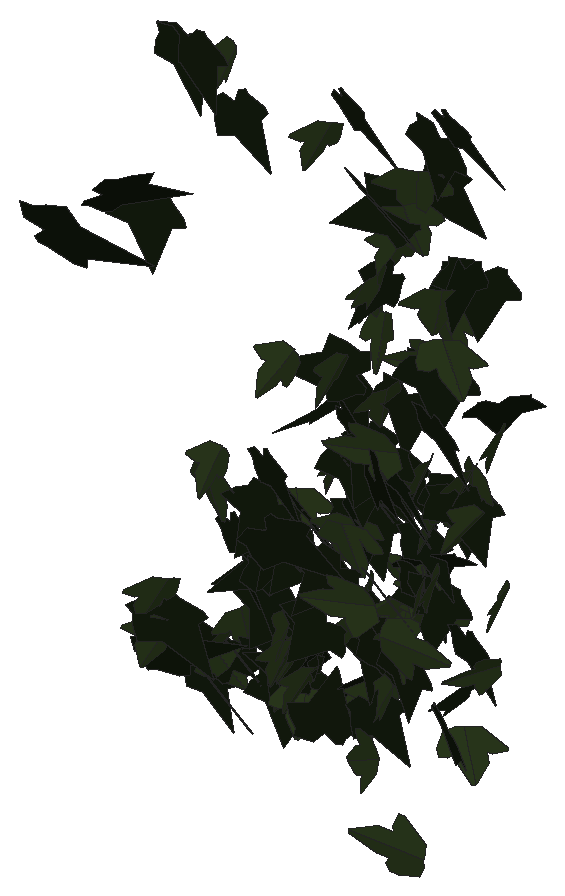
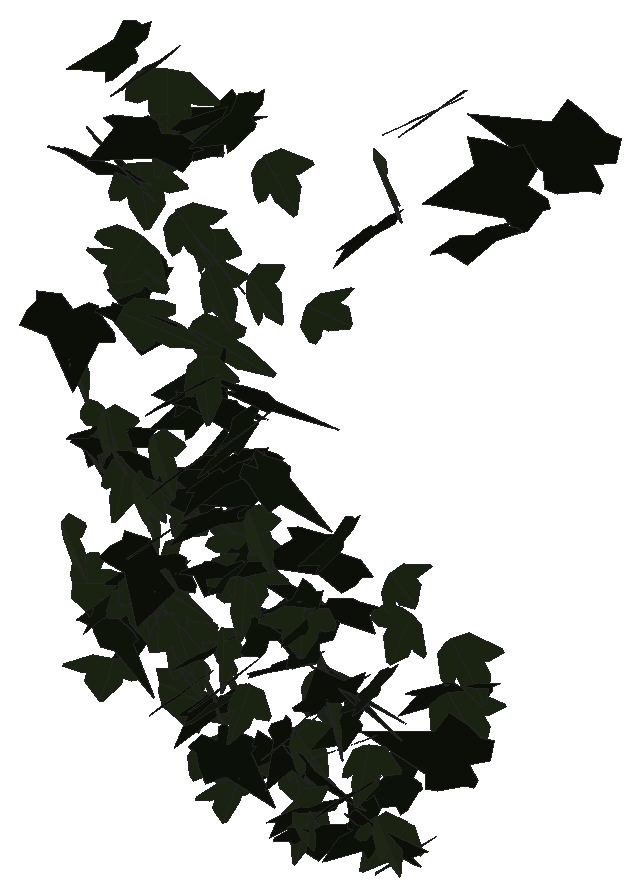
# SketchUp Ruby script. Lengths in inches.
U = 1.inch
M = Sketchup.active_model
def pt(a) = Geom::Point3d.new(a.map { |v| v * U })
def face(e, loops, mat)
  f = e.add_face(loops[0].map { |a| pt(a) })
  loops[1..].each { |l| e.add_face(l.map { |a| pt(a) }).erase! }
  f.material = f.back_material = mat if mat
  f
end
# faces: each face lists its corners as indices into pts; further lists are holes
def faces(e, pts, list, mat = nil) = list.each { |f| face(e, (f[0].is_a?(Array) ? f : [f]).map { |l| l.map { |i| pts[i] } }, mat) }
# xy, xz, yz: faces in a plane at the given z, y or x. An outline is a flat list of corners, or four numbers for a rectangle; further outlines are holes
def ring(l) = l.size == 4 ? [[l[0], l[1]], [l[2], l[1]], [l[2], l[3]], [l[0], l[3]]] : l.each_slice(2).to_a
def flat(e, list, mat, &to3) = list.each { |f| face(e, (f[0].is_a?(Array) ? f : [f]).map { |l| ring(l).map { |u, v| to3.(u, v) } }, mat) }
def xy(e, z, list, mat = nil) = flat(e, list, mat) { |x, y| [x, y, z] }
def xz(e, y, list, mat = nil) = flat(e, list, mat) { |x, z| [x, y, z] }
def yz(e, x, list, mat = nil) = flat(e, list, mat) { |y, z| [x, y, z] }
def lines(e, pts, list) = list.each { |a, b| e.add_line(pt(pts[a]), pt(pts[b])) }
# prism: a flat outline (further loops are holes) pulled along v
def prism(e, loops, v, mat = nil)
  f = face(e, loops, mat); d = Geom::Vector3d.new(v.map { |x| x * U })
  f.pushpull(f.normal.samedirection?(d) ? d.length : -d.length)
end
def box(e, o, s, mat = nil) = prism(e, [[o, [o[0] + s[0], o[1], o[2]], [o[0] + s[0], o[1] + s[1], o[2]], [o[0], o[1] + s[1], o[2]]]], [0, 0, s[2]], mat)
def at(x, y, z, deg = 0) = Geom::Transformation.translation(pt([x, y, z])) * Geom::Transformation.rotation(ORIGIN, Z_AXIS, deg.degrees)
def axes(o, x, y, z) = Geom::Transformation.new([*x, 0, *y, 0, *z, 0, *pt(o).to_a, 1])
def part(name) = M.definitions.add(name)
# library, detail: a bought-in or finely detailed component or shape, given as its bounding box
def library(name, o, s) = part(name).tap { |d| box(d.entities, o, s) }
def detail(e, o, s) = box(e.add_group.entities, o, s)
def put(e, d, t, mat = nil) = e.add_instance(d, t).tap { |i| i.material = mat if mat }
def group(e, t, mat = nil) = e.add_group.tap { |g| g.transformation = t; g.material = mat if mat }.entities
root = M.entities
M.materials.add("1026 AP 7946 SUNNY SIDE UP").color = [254, 231, 186]
M.materials.add("efeu1").color = [18, 25, 13]
M.materials.add("efeu2").color = [43, 57, 29]
c1 = part("ivyleaf_10")
p = [[0,0.5,-0.03],[-0.0625,2.02,-0.43],[-0.19,2.01,-0.46],[-0.54,1.05,-0.29],[-0.52,0.625,-0.18],[-0.83,0.76,-0.28],
  [-1.16,0.64,-0.33],[-1.15,0.33,-0.24],[-0.77,-0.39,0.02],[-0.3,-0.51,0.16],[0.04,-0.48,0.23],[-0.02,2.01,-0.4375],
  [-0.06,2.01,-0.43],[0.04,-0.49,0.23],[0.67,-0.49,0.14],[1.38,0.36,-0.2],[1.375,0.51,-0.24],[0.81,0.65,-0.19],
  [0.62,0.59,-0.15],[0.6,1.09,-0.28],[0.5,1.23,-0.31]]
faces(c1.entities,p,[[0,1,2,3,4,5,6,7,8,9,10],[11,12,0,13,14,15,16,17,18,19,20]],"efeu2")
c2 = part("ivyleaf_9")
p = [[1.54,2.16,1.25],[1.36,2.04,1.19],[-0.21,0.99,0.68],[-0.71,1.11,0.82],[-0.85,0.86,0.67],[-0.8,0.17,0.21],
  [-0.9,-0.01,0.1],[-0.67,-0.16,-0.02],[-0.08,-0.08,-0.05],[-0.03,-0.6,-0.4],[0.65,-0.88,-0.66],[0.83,-0.6,-0.49],
  [1.29,-0.42,-0.43],[1.8125,-0.07,-0.26],[1.21,0.44,0.15]]
faces(c2.entities,p,[[0,1,2,3,4,5,6,7,8,9,10,11,12,13,14]],"efeu1")
put(root,c1,axes([100.4,212.9375,280.08],[0.04345,-0.30572,0.04856],[-0.00086,-0.04912,-0.31648],[0.48681,0.0272,-0.0049]),"1026 AP 7946 SUNNY SIDE UP")
put(root,c1,axes([100.4,212.96,290.27],[0.30495,-0.28987,0.00995],[-0.00585,-0.01609,-0.35918],[0.45611,0.1936,-0.01126]),"1026 AP 7946 SUNNY SIDE UP")
put(root,c2,axes([100.73,212.63,279.72],[0.02636,0.13505,0.28405],[-0.34904,0.19485,-0.0912],[-0.36179,-0.17815,0.10868]),"1026 AP 7946 SUNNY SIDE UP")
put(root,c2,axes([100.32,211.1,288.47],[-0.12264,-0.34292,-0.04501],[0.01448,0.04072,-0.36206],[0.543,-0.07854,-0.00051]),"1026 AP 7946 SUNNY SIDE UP")
put(root,c2,axes([100.25,212.03,290.83],[0.05539,-0.34177,0.02697],[-0.01052,-0.03036,-0.36785],[0.58225,0.03196,-0.00921]),"1026 AP 7946 SUNNY SIDE UP")
put(root,c1,axes([100.46,212.44,283.04],[-0.46721,0.14937,-0.03435],[0.03162,-0.03683,-0.33483],[-0.25814,-0.27487,0.02115]),"1026 AP 7946 SUNNY SIDE UP")
put(root,c2,axes([100.18,210.23,288.93],[0.38363,0.15905,0.3046],[0.37128,0.1793,-0.29294],[-0.40612,0.31416,0.01992]),"1026 AP 7946 SUNNY SIDE UP")
put(root,c2,axes([100.29,212.53,279.58],[0.10473,-0.28789,-0.03038],[0.01787,0.0274,-0.31436],[0.49016,0.06051,0.01795]),"1026 AP 7946 SUNNY SIDE UP")
put(root,c2,axes([100.28,212.16,290.84],[0.03026,-0.35208,-0.00575],[0.06063,0.00258,-0.37543],[0.59459,0.01765,0.03857]),"1026 AP 7946 SUNNY SIDE UP")
put(root,c1,axes([100.66,211.05,281.08],[-0.2808,-0.26899,0.13538],[-0.05383,-0.13191,-0.33733],[0.50426,-0.16387,0.03938]),"1026 AP 7946 SUNNY SIDE UP")
put(root,c1,axes([100.66,210.97,281.86],[-0.16565,-0.31781,0.09898],[-0.04842,-0.09229,-0.3572],[0.56178,-0.10166,-0.0016]),"1026 AP 7946 SUNNY SIDE UP")
put(root,c2,axes([100.05,208.98,288.78],[0.33682,-0.06704,0.37385],[0.54164,-0.14519,-0.2254],[0.26971,0.37529,-0.01422]),"1026 AP 7946 SUNNY SIDE UP")
put(root,c1,axes([100.65,212.32,283.56],[-0.12589,-0.23386,0.2105],[0.1102,-0.21267,-0.24382],[0.51023,-0.01177,0.10459]),"1026 AP 7946 SUNNY SIDE UP")
put(root,c1,axes([100.58,212.57,279.86],[-0.25803,-0.23513,-0.15314],[0.19786,0.08948,-0.291],[0.38885,-0.20156,0.04645]),"1026 AP 7946 SUNNY SIDE UP")
put(root,c2,axes([100.5,213.03,289.39],[0.13506,-0.30745,-0.13915],[-0.05248,0.12911,-0.3281],[0.52432,0.09212,0.00301]),"1026 AP 7946 SUNNY SIDE UP")
put(root,c2,axes([100.34,211.27,280.41],[0.16045,0.03062,0.35834],[0.55402,0.073,-0.10493],[-0.13354,0.33966,-0.00476]),"1026 AP 7946 SUNNY SIDE UP")
put(root,c2,axes([100.64,212.77,282.13],[0.26445,-0.26633,-0.06387],[-0.03983,0.05552,-0.32406],[0.42759,0.16989,0.00931]),"1026 AP 7946 SUNNY SIDE UP")
put(root,c2,axes([100.62,211.07,281.39],[0.04734,-0.29086,-0.19688],[0.13483,0.18127,-0.2977],[0.56487,-0.01889,0.08756]),"1026 AP 7946 SUNNY SIDE UP")
put(root,c2,axes([100.8,212.6875,279.93],[0.41599,-0.15403,-0.05376],[-0.08799,0.00558,-0.31445],[0.23964,0.26943,-0.02213]),"1026 AP 7946 SUNNY SIDE UP")
put(root,c1,axes([101,212.52,280.8],[-0.1575,-0.29973,-0.08628],[0.11486,0.06108,-0.32138],[0.47495,-0.11416,0.04911]),"1026 AP 7946 SUNNY SIDE UP")
put(root,c2,axes([100.9,212.95,280.5],[0.18035,-0.26193,-0.13354],[-0.01525,0.13419,-0.29075],[0.45825,0.10755,0.04288]),"1026 AP 7946 SUNNY SIDE UP")
put(root,c2,axes([100.97,211.66,280.125],[0.42689,-0.17733,-0.03006],[-0.05072,0.00207,-0.33365],[0.27774,0.27294,-0.01473]),"1026 AP 7946 SUNNY SIDE UP")
put(root,c1,axes([101.28,212.95,281.63],[0.18206,-0.29358,-0.0409],[0.00022,0.0409,-0.3245],[0.46548,0.1148,0.01615]),"1026 AP 7946 SUNNY SIDE UP")
put(root,c2,axes([101.54,212.56,281.875],[-0.40653,0.18611,-0.01222],[-0.02452,-0.04355,-0.32523],[-0.29232,-0.25517,0.04427]),"1026 AP 7946 SUNNY SIDE UP")
put(root,c2,axes([101.36,212.93,281.74],[-0.25979,-0.11452,0.25359],[0.28172,0.17151,0.20655],[-0.32197,0.24248,-0.02388]),"1026 AP 7946 SUNNY SIDE UP")
put(root,c2,axes([101.625,212.57,281.84],[-0.48575,0.07752,-0.0144],[-0.01795,-0.10166,-0.31168],[-0.12267,-0.29207,0.10262]),"1026 AP 7946 SUNNY SIDE UP")
put(root,c2,axes([101.17,212.58,281.36],[0.34008,-0.22969,-0.03244],[-0.06441,0.00273,-0.32374],[0.35853,0.21836,-0.02739]),"1026 AP 7946 SUNNY SIDE UP")
put(root,c2,axes([101.41,212.88,280.9],[-0.22708,-0.23651,0.1531],[-0.0135,-0.1649,-0.27742],[0.44013,-0.12708,0.07047]),"1026 AP 7946 SUNNY SIDE UP")
put(root,c2,axes([101.67,212.54,282.94],[-0.40883,-0.21039,0.02359],[-0.00413,-0.03495,-0.34377],[0.33295,-0.25877,0.02471]),"1026 AP 7946 SUNNY SIDE UP")
put(root,c2,axes([101.52,212.58,281.6],[-0.00876,-0.30997,0.07029],[-0.01396,-0.06982,-0.3197],[0.49948,-0.00739,-0.0077]),"1026 AP 7946 SUNNY SIDE UP")
put(root,c2,axes([101.65,212.89,279.61],[-0.23227,-0.26827,-0.06348],[0.05461,0.04946,-0.31513],[0.42881,-0.15161,0.00575]),"1026 AP 7946 SUNNY SIDE UP")
put(root,c1,axes([101.83,212.87,279.88],[0.02513,-0.23873,0.20745],[0.04162,-0.20123,-0.24746],[0.49071,0.0293,0.01037]),"1026 AP 7946 SUNNY SIDE UP")
put(root,c1,axes([101.77,212.95,282.91],[0.33484,0.24255,0.01555],[-0.03056,0.03518,-0.33002],[-0.38077,0.21047,0.04015]),"1026 AP 7946 SUNNY SIDE UP")
put(root,c1,axes([101.89,212.82,279.65],[-0.37421,0.19947,0.01999],[-0.04411,-0.0051,-0.31913],[-0.31185,-0.23863,0.02116]),"1026 AP 7946 SUNNY SIDE UP")
put(root,c2,axes([101.64,212.3125,283.83],[0.26866,-0.29184,-0.01138],[-0.03436,-0.00193,-0.3478],[0.45784,0.1711,-0.01942]),"1026 AP 7946 SUNNY SIDE UP")
put(root,c2,axes([102.33,212.42,280.24],[-0.27344,0.16189,0.21147],[-0.25844,0.1226,-0.24343],[-0.31822,-0.23868,0.01599]),"1026 AP 7946 SUNNY SIDE UP")
put(root,c2,axes([101.76,212.88,279.91],[0.04147,-0.28781,-0.12595],[0.04682,0.12282,-0.29448],[0.48845,0.01266,0.03892]),"1026 AP 7946 SUNNY SIDE UP")
put(root,c2,axes([101.77,212.93,282.9],[0.29102,-0.24281,0.10729],[0.07688,-0.09519,-0.31454],[0.40913,0.1906,-0.01721]),"1026 AP 7946 SUNNY SIDE UP")
put(root,c1,axes([102.13,212.51,280.68],[0.00005,-0.29687,0.15007],[0.02015,-0.14724,-0.30647],[0.52075,0.00572,0.01184]),"1026 AP 7946 SUNNY SIDE UP")
put(root,c2,axes([102.06,212.875,280.91],[0.01062,-0.30476,0.08765],[-0.01617,-0.08699,-0.31431],[0.498,0.00367,-0.01208]),"1026 AP 7946 SUNNY SIDE UP")
put(root,c1,axes([102.32,212.93,289.61],[-0.14114,-0.31348,0.12088],[-0.0181,-0.12035,-0.33595],[0.527,-0.08809,0.02083]),"1026 AP 7946 SUNNY SIDE UP")
put(root,c2,axes([102.54,212.89,284.86],[-0.32656,0.21396,-0.14509],[0.01093,-0.17793,-0.28762],[-0.40368,-0.17791,0.10958]),"1026 AP 7946 SUNNY SIDE UP")
put(root,c2,axes([101.98,212.41,282.2],[0.24084,-0.22599,0.19939],[0.19396,-0.15145,-0.28177],[0.42721,0.19617,0.01552]),"1026 AP 7946 SUNNY SIDE UP")
put(root,c2,axes([102.45,212.36,280.55],[-0.06948,0.03479,-0.31981],[-0.28569,0.25242,0.05723],[0.39993,0.18636,-0.01468]),"1026 AP 7946 SUNNY SIDE UP")
put(root,c2,axes([102.44,212.45,282.52],[-0.32869,-0.24334,0.10703],[-0.06026,-0.10492,-0.32885],[0.41253,-0.20922,0.03724]),"1026 AP 7946 SUNNY SIDE UP")
put(root,c1,axes([102.4375,211.73,281.38],[0.24056,-0.27942,-0.10098],[-0.05703,0.09002,-0.32746],[0.46129,0.15685,0.01217]),"1026 AP 7946 SUNNY SIDE UP")
put(root,c1,axes([102.48,212.27,280.35],[-0.01962,-0.30415,0.13048],[-0.01494,-0.12809,-0.31432],[0.5189,-0.01519,-0.00412]),"1026 AP 7946 SUNNY SIDE UP")
put(root,c1,axes([102.49,211.75,281.0625],[-0.06248,-0.32051,0.07566],[0.01292,-0.07675,-0.33269],[0.51751,-0.03678,0.01744]),"1026 AP 7946 SUNNY SIDE UP")
put(root,c1,axes([102.44,212.26,279.95],[0.46693,0.10729,-0.00839],[0.00213,-0.02939,-0.32415],[-0.16925,0.29562,-0.02721]),"1026 AP 7946 SUNNY SIDE UP")
put(root,c1,axes([102.66,212.875,283.99],[0.04893,-0.32672,0.0268],[-0.00091,-0.02804,-0.33826],[0.51561,0.03096,-0.00314]),"1026 AP 7946 SUNNY SIDE UP")
put(root,c2,axes([102.3,211.6,283.1],[0.05122,-0.06588,-0.34066],[0.31779,0.26929,-0.03322],[0.42366,-0.19403,0.0661]),"1026 AP 7946 SUNNY SIDE UP")
put(root,c2,axes([102.4,212.93,282.35],[0.076,-0.21417,0.24091],[0.13452,-0.22024,-0.22613],[0.48159,0.09532,0.02515]),"1026 AP 7946 SUNNY SIDE UP")
put(root,c2,axes([103.11,212.61,285.73],[-0.39057,0.10536,0.20352],[-0.33228,-0.01541,-0.26615],[-0.1138,-0.31663,0.07861]),"1026 AP 7946 SUNNY SIDE UP")
put(root,c1,axes([102.85,211.28,286.5],[-0.13913,-0.18428,0.29259],[0.06511,-0.29824,-0.18713],[0.52975,-0.01174,0.09984]),"1026 AP 7946 SUNNY SIDE UP")
put(root,c2,axes([102.87,212.23,281.43],[-0.2707,-0.22697,0.15138],[-0.06465,-0.1517,-0.28938],[0.42133,-0.16911,0.05286]),"1026 AP 7946 SUNNY SIDE UP")
put(root,c1,axes([102.85,212.8,281.21],[-0.07735,-0.26194,-0.18395],[0.11246,0.16534,-0.27147],[0.48426,-0.08024,0.03366]),"1026 AP 7946 SUNNY SIDE UP")
put(root,c1,axes([103,212.76,282.79],[-0.41824,0.16926,0.07896],[-0.12535,0.0151,-0.32331],[-0.26322,-0.27614,0.0285]),"1026 AP 7946 SUNNY SIDE UP")
put(root,c2,axes([102.74,212.93,285.46],[0.10136,-0.32678,0.00248],[-0.00225,-0.00463,-0.34316],[0.51388,0.06444,-0.00199]),"1026 AP 7946 SUNNY SIDE UP")
put(root,c1,axes([103.12,212.63,283.05],[-0.43091,-0.16275,0.0669],[-0.06703,-0.05676,-0.32755],[0.26781,-0.27607,0.02566]),"1026 AP 7946 SUNNY SIDE UP")
put(root,c2,axes([102.73,212.94,290.26],[0.37878,-0.25121,-0.03896],[-0.02843,0.03306,-0.35822],[0.39812,0.24137,0.01149]),"1026 AP 7946 SUNNY SIDE UP")
put(root,c2,axes([103.03,212.05,279.68],[-0.3192,-0.10595,0.24116],[0.31593,0.12175,0.23636],[-0.25324,0.28543,-0.0091]),"1026 AP 7946 SUNNY SIDE UP")
put(root,c2,axes([103.31,212.83,280.35],[-0.14128,0.23304,-0.20031],[-0.00204,-0.2044,-0.25125],[-0.47855,-0.06793,0.0602]),"1026 AP 7946 SUNNY SIDE UP")
put(root,c1,axes([103.06,212.84,279.79],[0.16212,0.29753,0.01095],[0.00648,0.00803,-0.32434],[-0.468,0.10318,-0.0007]),"1026 AP 7946 SUNNY SIDE UP")
put(root,c2,axes([103.32,212,282.64],[-0.49417,-0.05569,-0.05445],[0.09211,-0.03201,-0.32625],[0.0775,-0.31703,0.04058]),"1026 AP 7946 SUNNY SIDE UP")
put(root,c1,axes([103.25,212.78,281.93],[0.04144,-0.29519,-0.1348],[0.03196,0.13087,-0.30306],[0.50564,0.01592,0.0302]),"1026 AP 7946 SUNNY SIDE UP")
put(root,c2,axes([103.14,212.9,283.18],[-0.1333,-0.28626,-0.13607],[0.10633,0.11537,-0.3054],[0.4831,-0.10438,0.02968]),"1026 AP 7946 SUNNY SIDE UP")
put(root,c2,axes([103.1,212.87,283.04],[0.04065,-0.22447,0.23974],[0.03702,-0.23281,-0.23413],[0.5085,0.03489,-0.00212]),"1026 AP 7946 SUNNY SIDE UP")
put(root,c2,axes([103.14,212.41,285.17],[0.37918,-0.1798,-0.18082],[-0.18963,0.12899,-0.30787],[0.34533,0.26826,0.02948]),"1026 AP 7946 SUNNY SIDE UP")
put(root,c1,axes([103.28,212.3,283.12],[-0.49797,0.0196,-0.07446],[0.10537,-0.0671,-0.32113],[-0.05294,-0.31786,0.06124]),"1026 AP 7946 SUNNY SIDE UP")
put(root,c2,axes([103.03,212.45,284.34],[0.42302,-0.21437,0.0263],[0.00762,-0.03672,-0.35361],[0.3396,0.26785,-0.02483]),"1026 AP 7946 SUNNY SIDE UP")
put(root,c2,axes([103.56,212.83,280.9375],[-0.11569,-0.30104,0.08003],[0.01744,0.07899,0.31962],[-0.48923,0.074,-0.00753]),"1026 AP 7946 SUNNY SIDE UP")
put(root,c2,axes([103.22,212.875,284.57],[0.10706,-0.27277,-0.18208],[-0.06697,0.16994,-0.28863],[0.50533,0.08031,0.00033]),"1026 AP 7946 SUNNY SIDE UP")
put(root,c1,axes([103.48,212.84,280.17],[-0.19926,-0.25257,0.1437],[-0.00121,-0.15356,-0.28514],[0.45477,-0.11107,0.0622]),"1026 AP 7946 SUNNY SIDE UP")
put(root,c1,axes([103.47,212.73,287.39],[-0.03806,-0.33276,0.06584],[0.00779,-0.0663,-0.34396],[0.53331,-0.02278,0.00972]),"1026 AP 7946 SUNNY SIDE UP")
put(root,c2,axes([103.2,212.92,283.99],[0.10226,-0.25809,-0.19981],[0.04142,0.19998,-0.26589],[0.50456,0.03589,0.06232]),"1026 AP 7946 SUNNY SIDE UP")
put(root,c2,axes([103.48,212.82,280.8],[-0.09026,-0.26831,0.16658],[0.00608,-0.16652,-0.28157],[0.49379,-0.04699,0.03392]),"1026 AP 7946 SUNNY SIDE UP")
put(root,c2,axes([103.51,212.36,284.5],[-0.19687,-0.31774,-0.0619],[0.06113,0.04723,-0.35104],[0.50426,-0.12978,0.01839]),"1026 AP 7946 SUNNY SIDE UP")
put(root,c2,axes([103.53,212.83,281.7],[0.02937,-0.31863,-0.02625],[0.01475,0.02425,-0.32848],[0.50217,0.01792,0.01118]),"1026 AP 7946 SUNNY SIDE UP")
put(root,c1,axes([103.75,211.45,286.65],[0.03859,-0.30404,0.18162],[0.05266,-0.17564,-0.3148],[0.55149,0.03804,0.01735]),"1026 AP 7946 SUNNY SIDE UP")
put(root,c1,axes([103.84,212.91,288.25],[-0.16035,-0.28674,0.16282],[-0.00732,-0.16593,-0.311],[0.51602,-0.09146,0.04618]),"1026 AP 7946 SUNNY SIDE UP")
put(root,c1,axes([103.77,212.375,287.69],[-0.01957,-0.34731,-0.07493],[0.08904,0.06795,-0.35344],[0.55018,-0.02335,0.05453]),"1026 AP 7946 SUNNY SIDE UP")
put(root,c2,axes([103.93,212.51,287.79],[-0.45581,0.08793,-0.16313],[0.22059,-0.08148,-0.31069],[-0.18122,-0.32035,0.03211]),"1026 AP 7946 SUNNY SIDE UP")
put(root,c1,axes([103.88,212.45,285.72],[-0.11139,-0.32433,-0.04358],[0.01659,0.03911,-0.34176],[0.51366,-0.07159,0.00159]),"1026 AP 7946 SUNNY SIDE UP")
put(root,c1,axes([104.1875,212.83,282.34],[0.09152,0.0268,0.32907],[-0.49348,0.07009,0.05329],[-0.10141,-0.31688,0.03766]),"1026 AP 7946 SUNNY SIDE UP")
put(root,c1,axes([104.28,211.31,282.66],[0.19388,-0.04593,-0.34283],[-0.51826,0.05054,-0.1328],[0.09998,0.35102,-0.02361]),"1026 AP 7946 SUNNY SIDE UP")
put(root,c1,axes([104.02,212.74,281.52],[-0.06119,-0.3082,0.07462],[-0.01647,-0.07345,-0.32045],[0.49818,-0.04028,-0.00143]),"1026 AP 7946 SUNNY SIDE UP")
put(root,c1,axes([104.03,212.82,281.93],[-0.16261,-0.30525,0.03647],[-0.00378,-0.03837,-0.33209],[0.48351,-0.10296,0.00967]),"1026 AP 7946 SUNNY SIDE UP")
put(root,c1,axes([104.03,212.81,281.84],[-0.33116,-0.2374,0.06375],[0.0267,-0.09715,-0.31808],[0.38538,-0.19727,0.07682]),"1026 AP 7946 SUNNY SIDE UP")
put(root,c1,axes([103.9,212.34,287.02],[0.38612,-0.1916,0.17491],[0.18516,-0.12605,-0.32069],[0.35871,0.27131,-0.02274]),"1026 AP 7946 SUNNY SIDE UP")
put(root,c2,axes([103.98,212.89,285.51],[-0.07231,-0.3188,0.09151],[-0.00066,-0.09145,-0.33213],[0.52115,-0.04435,0.01227]),"1026 AP 7946 SUNNY SIDE UP")
put(root,c2,axes([104.16,212.06,285],[-0.42651,-0.18313,-0.06183],[0.10546,0.00554,-0.33547],[0.28354,-0.27753,0.03177]),"1026 AP 7946 SUNNY SIDE UP")
put(root,c2,axes([103.92,212.8125,284.38],[0.16464,-0.29967,-0.09595],[-0.02826,0.0905,-0.32624],[0.49184,0.10552,0.01337]),"1026 AP 7946 SUNNY SIDE UP")
put(root,c2,axes([103.76,212.22,289.33],[0.21313,-0.2662,0.20553],[0.19233,-0.16221,-0.3072],[0.48799,0.1802,0.03131]),"1026 AP 7946 SUNNY SIDE UP")
put(root,c2,axes([103.98,212.05,280.45],[0.07989,-0.25939,-0.2106],[-0.06002,0.19934,-0.27113],[0.51438,0.06355,0.00108]),"1026 AP 7946 SUNNY SIDE UP")
put(root,c2,axes([104.01,212.83,280.875],[-0.01076,-0.30822,0.08156],[-0.0149,-0.08071,-0.31798],[0.50084,-0.00902,-0.00771]),"1026 AP 7946 SUNNY SIDE UP")
put(root,c2,axes([104.37,212.27,289.2],[-0.3024,-0.12163,0.28887],[-0.30089,-0.21144,-0.23036],[0.37603,-0.267,0.04797]),"1026 AP 7946 SUNNY SIDE UP")
put(root,c1,axes([104.22,212.04,280.76],[0.27049,-0.28678,-0.02061],[-0.03676,0.00738,-0.34407],[0.45036,0.17285,-0.0157]),"1026 AP 7946 SUNNY SIDE UP")
put(root,c1,axes([104.71,211.33,285.5],[0.199,-0.01979,-0.34829],[-0.52198,0.06355,-0.13153],[0.10446,0.35525,0.00628]),"1026 AP 7946 SUNNY SIDE UP")
put(root,c1,axes([104.41,212.75,284.48],[0.04076,-0.33222,0.01936],[0.00053,-0.02071,-0.34341],[0.52339,0.0259,-0.00116]),"1026 AP 7946 SUNNY SIDE UP")
put(root,c1,axes([104.72,212.8,286.41],[0.15299,0.02514,-0.33243],[-0.50768,-0.01814,-0.10181],[-0.03878,0.33669,0.02132]),"1026 AP 7946 SUNNY SIDE UP")
put(root,c2,axes([104.4,212.82,282.83],[0.31106,0.25918,-0.03034],[-0.05885,-0.01023,-0.33509],[-0.40619,0.19997,0.02532]),"1026 AP 7946 SUNNY SIDE UP")
put(root,c1,axes([104.43,212.79,282.31],[-0.06911,0.26788,-0.18375],[-0.06002,-0.18458,-0.27465],[-0.5038,-0.01476,0.05793]),"1026 AP 7946 SUNNY SIDE UP")
put(root,c2,axes([104.28,212.82,282.51],[0.13726,-0.31455,-0.0023],[-0.00309,-0.00008,-0.33629],[0.49459,0.08729,-0.00146]),"1026 AP 7946 SUNNY SIDE UP")
put(root,c1,axes([104.49,212.6,282.49],[0.14141,-0.2846,-0.13346],[0.05374,0.14132,-0.29831],[0.48769,0.06695,0.07157]),"1026 AP 7946 SUNNY SIDE UP")
put(root,c1,axes([104.46,212.27,289.18],[-0.39896,-0.23764,-0.0996],[0.16747,0.02409,-0.35376],[0.36612,-0.26997,0.05328]),"1026 AP 7946 SUNNY SIDE UP")
put(root,c2,axes([104.31,212.84,283.22],[0.13342,-0.31042,-0.06896],[-0.00804,0.06612,-0.3309],[0.49869,0.08412,0.01312]),"1026 AP 7946 SUNNY SIDE UP")
put(root,c1,axes([104.61,212.81,282.375],[-0.34937,-0.18643,0.15152],[-0.01746,-0.19428,-0.27018],[0.37401,-0.18322,0.12892]),"1026 AP 7946 SUNNY SIDE UP")
put(root,c1,axes([104.79,210.94,280.29],[0.17848,-0.20912,-0.29144],[-0.25425,0.23159,-0.24286],[0.48959,0.1965,-0.01988]),"1026 AP 7946 SUNNY SIDE UP")
put(root,c2,axes([104.28,212.9375,289.47],[-0.05405,-0.14434,-0.32535],[0.28085,0.26386,-0.1431],[0.46686,-0.17544,0.04842]),"1026 AP 7946 SUNNY SIDE UP")
put(root,c1,axes([104.65,212.3,289.84],[-0.45601,-0.22005,0.00416],[0.02278,-0.0278,-0.37385],[0.34536,-0.28872,0.03015]),"1026 AP 7946 SUNNY SIDE UP")
put(root,c1,axes([104.73,212.8,282.1],[-0.37185,-0.2096,0.07326],[-0.01309,-0.09724,-0.31903],[0.34838,-0.22737,0.0662]),"1026 AP 7946 SUNNY SIDE UP")
put(root,c1,axes([104.68,212.77,283.78],[0.07663,-0.27691,0.17956],[0.05979,-0.17183,-0.29058],[0.51233,0.06147,0.00705]),"1026 AP 7946 SUNNY SIDE UP")
put(root,c2,axes([104.6,212.91,290.25],[-0.04249,-0.31806,0.14874],[0.00067,-0.14665,-0.32948],[0.55042,-0.02437,0.01189]),"1026 AP 7946 SUNNY SIDE UP")
put(root,c2,axes([104.48,211.73,284.69],[0.36595,-0.23732,0.0021],[-0.02005,-0.01723,-0.34184],[0.37266,0.23212,-0.02045]),"1026 AP 7946 SUNNY SIDE UP")
put(root,c1,axes([104.6,211.98,281.93],[0.31799,-0.14744,0.23514],[0.27128,-0.15149,-0.25823],[0.33152,0.26538,-0.01423]),"1026 AP 7946 SUNNY SIDE UP")
put(root,c2,axes([104.74,212.6875,282.42],[-0.21356,-0.29096,-0.03833],[0.02806,0.0309,-0.3306],[0.46006,-0.13695,0.00238]),"1026 AP 7946 SUNNY SIDE UP")
put(root,c2,axes([104.47,211.36,285.14],[0.1175,-0.09563,-0.34819],[0.5294,-0.07709,0.09887],[-0.15449,-0.33691,0.07397]),"1026 AP 7946 SUNNY SIDE UP")
put(root,c2,axes([104.77,212.73,286.37],[-0.36874,-0.17554,-0.17446],[0.24058,0.07532,-0.30003],[0.2973,-0.27868,0.02641]),"1026 AP 7946 SUNNY SIDE UP")
put(root,c2,axes([104.57,211.71,284.95],[0.284,-0.27376,0.06012],[0.03201,-0.05827,-0.33787],[0.43948,0.18115,-0.01424]),"1026 AP 7946 SUNNY SIDE UP")
put(root,c1,axes([104.93,212.82,283.99],[-0.15438,-0.2907,-0.13311],[0.08103,0.11715,-0.31522],[0.49254,-0.11039,0.01014]),"1026 AP 7946 SUNNY SIDE UP")
put(root,c2,axes([104.93,211.3,282.89],[0.35193,-0.28521,0.0322],[-0.00304,0.04018,0.37297],[-0.45143,-0.22262,0.02259]),"1026 AP 7946 SUNNY SIDE UP")
put(root,c1,axes([104.89,212.67,287.4],[-0.5026,0.05833,-0.11119],[0.14573,-0.08389,-0.32896],[-0.1271,-0.32688,0.06249]),"1026 AP 7946 SUNNY SIDE UP")
put(root,c1,axes([104.88,211.98,282.2],[0.1383,-0.26091,0.20598],[0.15385,-0.17841,-0.28314],[0.49493,0.12837,0.03046]),"1026 AP 7946 SUNNY SIDE UP")
put(root,c2,axes([104.76,212.93,290.61],[0.36668,-0.2643,-0.00113],[0.03531,0.01927,-0.36172],[0.41409,0.2324,0.03184]),"1026 AP 7946 SUNNY SIDE UP")
put(root,c1,axes([105.16,212.05,283.07],[0.1193,-0.31528,-0.05317],[-0.00086,0.05108,-0.33357],[0.5019,0.07503,0.01207]),"1026 AP 7946 SUNNY SIDE UP")
put(root,c1,axes([105.21,212.8,284.59],[0.02071,-0.33214,0.0387],[-0.01674,-0.03988,-0.34244],[0.52566,0.01182,-0.01243]),"1026 AP 7946 SUNNY SIDE UP")
put(root,c2,axes([105.07,212.87,284.26],[-0.33332,-0.16382,-0.20409],[0.28583,0.08435,-0.27303],[0.28422,-0.27695,0.03523]),"1026 AP 7946 SUNNY SIDE UP")
put(root,c1,axes([105.28,212.08,288.08],[-0.31173,-0.28247,0.02429],[0.00211,-0.03165,-0.35515],[0.44591,-0.19732,0.01866]),"1026 AP 7946 SUNNY SIDE UP")
put(root,c1,axes([105.38,212.83,284.65],[-0.38674,0.22795,0.01902],[-0.10486,-0.04743,-0.33577],[-0.34382,-0.24195,0.08101]),"1026 AP 7946 SUNNY SIDE UP")
put(root,c1,axes([105.1,212.43,286.9],[0.47865,0.08014,0.13128],[0.19798,0.02016,-0.32394],[-0.12864,0.32921,-0.01007]),"1026 AP 7946 SUNNY SIDE UP")
put(root,c2,axes([105.65,212.29,281.16],[-0.23258,0.28809,-0.02144],[-0.00399,-0.02651,-0.33345],[-0.45436,-0.14724,0.0139]),"1026 AP 7946 SUNNY SIDE UP")
put(root,c2,axes([105.3,212.58,284.34],[-0.1346,-0.27701,-0.16849],[0.12159,0.14489,-0.29653],[0.4897,-0.11211,0.02732]),"1026 AP 7946 SUNNY SIDE UP")
put(root,c1,axes([105.94,210.5,279.2],[0.00678,0.05593,0.3893],[-0.59249,-0.0596,0.01318],[0.09572,-0.37286,0.054]),"1026 AP 7946 SUNNY SIDE UP")
put(root,c2,axes([105.28,212.73,281.76],[0.19495,-0.29617,0.02909],[-0.00748,-0.03438,-0.33047],[0.468,0.12282,-0.0174]),"1026 AP 7946 SUNNY SIDE UP")
put(root,c1,axes([105.57,212.5,284.1],[-0.02358,-0.21418,0.25912],[0.00647,-0.2531,-0.22219],[0.52088,-0.00655,0.01449]),"1026 AP 7946 SUNNY SIDE UP")
put(root,c2,axes([105.47,212.41,288.45],[-0.32786,-0.11395,-0.26069],[0.43455,-0.1059,-0.18656],[-0.02795,-0.30978,0.1574]),"1026 AP 7946 SUNNY SIDE UP")
put(root,c1,axes([105.25,211.03,282.47],[0.01561,-0.03966,-0.38335],[0.53561,-0.15263,0.02525],[-0.24279,-0.33927,0.03104]),"1026 AP 7946 SUNNY SIDE UP")
put(root,c2,axes([105.43,211.71,286.09],[0.21781,-0.30562,0.11253],[0.06553,-0.10293,-0.34625],[0.50704,0.14459,-0.00359]),"1026 AP 7946 SUNNY SIDE UP")
put(root,c2,axes([105.58,211.91,280.58],[0.02056,-0.16603,0.30892],[0.05648,-0.29872,-0.17321],[0.5373,0.03775,0.00638]),"1026 AP 7946 SUNNY SIDE UP")
put(root,c1,axes([105.83,212.8,285.5],[0.10551,-0.3311,-0.00717],[0.0084,0.00626,-0.34794],[0.52062,0.067,0.00706]),"1026 AP 7946 SUNNY SIDE UP")
put(root,c2,axes([105.87,212.8,286.09],[0.1901,0.30912,-0.07686],[-0.0197,-0.077,-0.34199],[-0.50028,0.1205,-0.01574]),"1026 AP 7946 SUNNY SIDE UP")
put(root,c2,axes([105.71,212.57,288.41],[-0.34683,-0.22791,-0.14332],[0.29971,-0.01007,-0.29714],[0.29253,-0.2599,0.13451]),"1026 AP 7946 SUNNY SIDE UP")
put(root,c1,axes([105.87,212.86,282.7],[0.14854,-0.3087,0.04035],[0.00928,-0.04098,-0.33276],[0.48957,0.09444,-0.00593]),"1026 AP 7946 SUNNY SIDE UP")
put(root,c1,axes([105.72,212.16,280.42],[0.36872,0.22452,0.0411],[0.0647,0.01277,-0.3338],[-0.35233,0.23731,-0.01829]),"1026 AP 7946 SUNNY SIDE UP")
put(root,c1,axes([106.05,212.33,281.67],[-0.08168,0.1009,-0.31275],[-0.31504,-0.25071,-0.05189],[-0.39327,0.17988,0.10653]),"1026 AP 7946 SUNNY SIDE UP")
